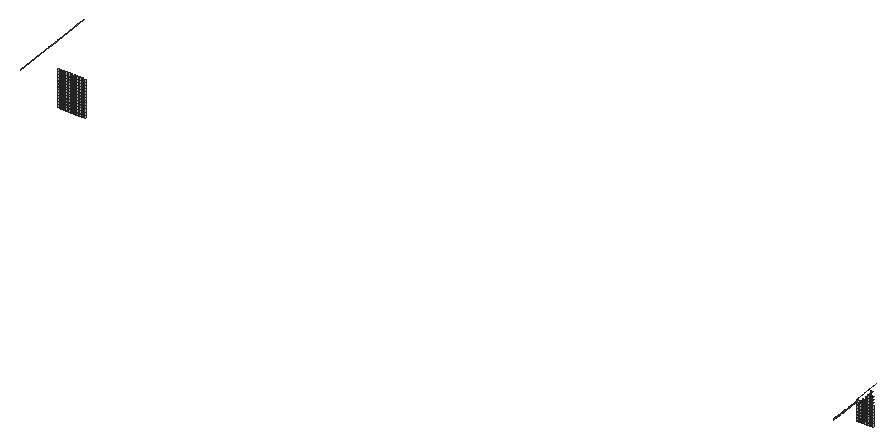
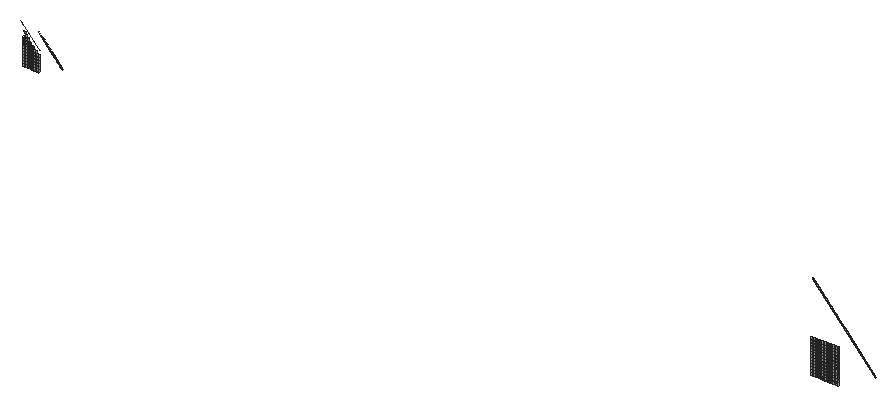
# SketchUp Ruby script. Lengths in inches.
U = 1.inch
M = Sketchup.active_model
def pt(a) = Geom::Point3d.new(a.map { |v| v * U })
def face(e, loops, mat)
  f = e.add_face(loops[0].map { |a| pt(a) })
  loops[1..].each { |l| e.add_face(l.map { |a| pt(a) }).erase! }
  f.material = f.back_material = mat if mat
  f
end
# faces: each face lists its corners as indices into pts; further lists are holes
def faces(e, pts, list, mat = nil) = list.each { |f| face(e, (f[0].is_a?(Array) ? f : [f]).map { |l| l.map { |i| pts[i] } }, mat) }
# xy, xz, yz: faces in a plane at the given z, y or x. An outline is a flat list of corners, or four numbers for a rectangle; further outlines are holes
def ring(l) = l.size == 4 ? [[l[0], l[1]], [l[2], l[1]], [l[2], l[3]], [l[0], l[3]]] : l.each_slice(2).to_a
def flat(e, list, mat, &to3) = list.each { |f| face(e, (f[0].is_a?(Array) ? f : [f]).map { |l| ring(l).map { |u, v| to3.(u, v) } }, mat) }
def xy(e, z, list, mat = nil) = flat(e, list, mat) { |x, y| [x, y, z] }
def xz(e, y, list, mat = nil) = flat(e, list, mat) { |x, z| [x, y, z] }
def yz(e, x, list, mat = nil) = flat(e, list, mat) { |y, z| [x, y, z] }
def lines(e, pts, list) = list.each { |a, b| e.add_line(pt(pts[a]), pt(pts[b])) }
# prism: a flat outline (further loops are holes) pulled along v
def prism(e, loops, v, mat = nil)
  f = face(e, loops, mat); d = Geom::Vector3d.new(v.map { |x| x * U })
  f.pushpull(f.normal.samedirection?(d) ? d.length : -d.length)
end
def box(e, o, s, mat = nil) = prism(e, [[o, [o[0] + s[0], o[1], o[2]], [o[0] + s[0], o[1] + s[1], o[2]], [o[0], o[1] + s[1], o[2]]]], [0, 0, s[2]], mat)
def at(x, y, z, deg = 0) = Geom::Transformation.translation(pt([x, y, z])) * Geom::Transformation.rotation(ORIGIN, Z_AXIS, deg.degrees)
def axes(o, x, y, z) = Geom::Transformation.new([*x, 0, *y, 0, *z, 0, *pt(o).to_a, 1])
def part(name) = M.definitions.add(name)
# library, detail: a bought-in or finely detailed component or shape, given as its bounding box
def library(name, o, s) = part(name).tap { |d| box(d.entities, o, s) }
def detail(e, o, s) = box(e.add_group.entities, o, s)
def put(e, d, t, mat = nil) = e.add_instance(d, t).tap { |i| i.material = mat if mat }
def group(e, t, mat = nil) = e.add_group.tap { |g| g.transformation = t; g.material = mat if mat }.entities
root = M.entities
M.materials.add("[Color M06]").color = [79, 71, 84]
xy(root,305.35,[[1357.49,480.14,1359.8,480.77],[1360.4,480.14,1362.71,480.77],[1363.3125,480.14,1365.625,480.77],[1366.23,480.14,1368.54,480.64],[1369.14,480.14,1371.45,480.64],
  [1372.05,480.14,1374.36,480.64],[1374.96,480.14,1377.27,480.64],[1377.875,480.14,1380.1875,480.77],[1380.79,480.14,1383.1,480.77],[1383.7,480.14,1386.01,480.77],
  [2206.1,480.14,2208.41,480.77],[2209.01,480.14,2211.32,480.77],[2211.92,480.14,2214.23,480.77],[2214.83,480.14,2217.15,480.77],[2217.75,480.14,2220.06,480.77],
  [2220.66,480.14,2222.97,480.77]])
xy(root,307.67,[[1357.49,480.14,1359.8,480.77],[1360.4,480.14,1362.71,480.77],[1363.3125,480.14,1365.625,480.77],[1366.23,480.14,1368.54,480.64],[1369.14,480.14,1371.45,480.64],
  [1372.05,480.14,1374.36,480.64],[1374.96,480.14,1377.27,480.64],[1377.875,480.14,1380.1875,480.77],[1380.79,480.14,1383.1,480.77],[1383.7,480.14,1386.01,480.77],
  [2206.1,480.14,2208.41,480.77],[2209.01,480.14,2211.32,480.77],[2211.92,480.14,2214.23,480.77],[2214.83,480.14,2217.15,480.77],[2217.75,480.14,2220.06,480.77],
  [2220.66,480.14,2222.97,480.77]])
xy(root,308.4,[[1357.52,480.14,1359.83,480.77],[1360.43,480.14,1362.74,480.77],[1363.34,480.14,1365.65,480.77],[1366.25,480.14,1368.57,480.77],[1369.17,480.14,1371.48,480.77],
  [1372.08,480.14,1374.39,480.77],[1374.99,480.14,1377.3,480.77],[1377.9,480.14,1380.22,480.77],[1380.81,480.14,1383.13,480.77],[1383.73,480.14,1386.04,480.77],
  [2206.125,480.14,2208.4375,480.77],[2209.04,480.14,2211.35,480.77],[2211.95,480.14,2214.26,480.77],[2214.86,480.14,2217.17,480.77],[2217.77,480.14,2220.09,480.77],
  [2220.6875,480.14,2223,480.77]])
xy(root,310.71,[[1357.52,480.14,1359.83,480.77],[1360.43,480.14,1362.74,480.77],[1363.34,480.14,1365.65,480.77],[1366.25,480.14,1368.57,480.77],[1369.17,480.14,1371.48,480.77],
  [1372.08,480.14,1374.39,480.77],[1374.99,480.14,1377.3,480.77],[1377.9,480.14,1380.22,480.77],[1380.81,480.14,1383.13,480.77],[1383.73,480.14,1386.04,480.77],
  [2206.125,480.14,2208.4375,480.77],[2209.04,480.14,2211.35,480.77],[2211.95,480.14,2214.26,480.77],[2214.86,480.14,2217.17,480.77],[2217.77,480.14,2220.09,480.77],
  [2220.6875,480.14,2223,480.77]])
xy(root,311.21,[[1357.52,480.14,1359.83,480.77],[1360.43,480.14,1362.74,480.77],[1363.34,480.14,1365.65,480.77],[1366.25,480.14,1368.57,480.77],[1369.17,480.14,1371.48,480.77],
  [1372.08,480.14,1374.39,480.77],[1374.99,480.14,1377.3,480.77],[1377.9,480.14,1380.22,480.77],[1380.81,480.14,1383.13,480.77],[1383.73,480.14,1386.04,480.77],
  [2206.125,480.14,2208.4375,480.77],[2209.04,480.14,2211.35,480.77],[2211.95,480.14,2214.26,480.77],[2214.86,480.14,2217.17,480.77],[2217.77,480.14,2220.09,480.77],
  [2220.6875,480.14,2223,480.77]])
xy(root,313.52,[[1357.52,480.14,1359.83,480.77],[1360.43,480.14,1362.74,480.77],[1363.34,480.14,1365.65,480.77],[1366.25,480.14,1368.57,480.77],[1369.17,480.14,1371.48,480.77],
  [1372.08,480.14,1374.39,480.77],[1374.99,480.14,1377.3,480.77],[1377.9,480.14,1380.22,480.77],[1380.81,480.14,1383.13,480.77],[1383.73,480.14,1386.04,480.77],
  [2206.125,480.14,2208.4375,480.77],[2209.04,480.14,2211.35,480.77],[2211.95,480.14,2214.26,480.77],[2214.86,480.14,2217.17,480.77],[2217.77,480.14,2220.09,480.77],
  [2220.6875,480.14,2223,480.77]])
xy(root,314.02,[[1357.52,480.14,1359.83,480.77],[1360.43,480.14,1362.74,480.77],[1363.34,480.14,1365.65,480.77],[1366.25,480.14,1368.57,480.77],[1369.17,480.14,1371.48,480.77],
  [1372.08,480.14,1374.39,480.77],[1374.99,480.14,1377.3,480.77],[1377.9,480.14,1380.22,480.77],[1380.81,480.14,1383.13,480.77],[1383.73,480.14,1386.04,480.77],
  [2206.125,480.14,2208.4375,480.77],[2209.04,480.14,2211.35,480.77],[2211.95,480.14,2214.26,480.77],[2214.86,480.14,2217.17,480.77],[2217.77,480.14,2220.09,480.77],
  [2220.6875,480.14,2223,480.77]])
xy(root,316.34,[[1357.52,480.14,1359.83,480.77],[1360.43,480.14,1362.74,480.77],[1363.34,480.14,1365.65,480.77],[1366.25,480.14,1368.57,480.77],[1369.17,480.14,1371.48,480.77],
  [1372.08,480.14,1374.39,480.77],[1374.99,480.14,1377.3,480.77],[1377.9,480.14,1380.22,480.77],[1380.81,480.14,1383.13,480.77],[1383.73,480.14,1386.04,480.77],
  [2206.125,480.14,2208.4375,480.77],[2209.04,480.14,2211.35,480.77],[2211.95,480.14,2214.26,480.77],[2214.86,480.14,2217.17,480.77],[2217.77,480.14,2220.09,480.77],
  [2220.6875,480.14,2223,480.77]])
xy(root,316.84,[[1357.52,480.14,1359.83,480.77],[1360.43,480.14,1362.74,480.77],[1363.34,480.14,1365.65,480.77],[1366.25,480.14,1368.57,480.77],[1369.17,480.14,1371.48,480.77],
  [1372.08,480.14,1374.39,480.77],[1374.99,480.14,1377.3,480.77],[1377.9,480.14,1380.22,480.77],[1380.81,480.14,1383.13,480.77],[1383.73,480.14,1386.04,480.77],
  [2206.125,480.14,2208.4375,480.77],[2209.04,480.14,2211.35,480.77],[2211.95,480.14,2214.26,480.77],[2214.86,480.14,2217.17,480.77],[2217.77,480.14,2220.09,480.77],
  [2220.6875,480.14,2223,480.77]])
xy(root,319.15,[[1357.52,480.14,1359.83,480.77],[1360.43,480.14,1362.74,480.77],[1363.34,480.14,1365.65,480.77],[1366.25,480.14,1368.57,480.77],[1369.17,480.14,1371.48,480.77],
  [1372.08,480.14,1374.39,480.77],[1374.99,480.14,1377.3,480.77],[1377.9,480.14,1380.22,480.77],[1380.81,480.14,1383.13,480.77],[1383.73,480.14,1386.04,480.77],
  [2206.125,480.14,2208.4375,480.77],[2209.04,480.14,2211.35,480.77],[2211.95,480.14,2214.26,480.77],[2214.86,480.14,2217.17,480.77],[2217.77,480.14,2220.09,480.77],
  [2220.6875,480.14,2223,480.77]])
xy(root,319.65,[[1357.52,480.14,1359.83,480.77],[1360.43,480.14,1362.74,480.77],[1363.34,480.14,1365.65,480.77],[1366.25,480.14,1368.57,480.77],[1369.17,480.14,1371.48,480.77],
  [1372.08,480.14,1374.39,480.7],[1374.99,480.14,1377.3,480.7],[1377.9,480.14,1380.22,480.7],[1380.81,480.14,1383.13,480.7],[1383.73,480.14,1386.04,480.77],
  [2206.125,480.14,2208.4375,480.77],[2209.04,480.14,2211.35,480.77],[2211.95,480.14,2214.26,480.77],[2214.86,480.14,2217.17,480.77],[2217.77,480.14,2220.09,480.77],
  [2220.6875,480.14,2223,480.77]])
xy(root,321.96,[[1357.52,480.14,1359.83,480.77],[1360.43,480.14,1362.74,480.77],[1363.34,480.14,1365.65,480.77],[1366.25,480.14,1368.57,480.77],[1369.17,480.14,1371.48,480.77],
  [1372.08,480.14,1374.39,480.7],[1374.99,480.14,1377.3,480.7],[1377.9,480.14,1380.22,480.7],[1380.81,480.14,1383.13,480.7],[1383.73,480.14,1386.04,480.77],
  [2206.66,480.14,2208.4375,480.77],[2209.04,480.14,2211.35,480.77],[2211.95,480.14,2214.26,480.77],[2214.86,480.14,2217.17,480.77],[2217.77,480.14,2220.09,480.77],
  [2220.6875,480.14,2223,480.77]])
xy(root,322.46,[[1357.52,480.14,1359.83,480.77],[1360.43,480.14,1362.74,480.77],[1363.34,480.14,1365.65,480.77],[1366.25,480.14,1368.57,480.77],[1369.17,480.14,1371.48,480.77],
  [1372.08,480.14,1374.39,480.77],[1374.99,480.14,1377.3,480.77],[1377.9,480.14,1380.22,480.77],[1380.81,480.14,1383.13,480.77],[1383.73,480.14,1386.04,480.77],
  [2209.04,480.14,2211.35,480.77],[2211.95,480.14,2214.26,480.77],[2214.86,480.14,2217.17,480.77],[2217.77,480.14,2220.09,480.77],[2220.6875,480.14,2223,480.77]])
xy(root,324.77,[[1357.52,480.14,1359.83,480.77],[1360.43,480.14,1362.74,480.77],[1363.34,480.14,1365.65,480.77],[1366.25,480.14,1368.57,480.77],[1369.17,480.14,1371.48,480.77],
  [1372.08,480.14,1374.39,480.77],[1374.99,480.14,1377.3,480.77],[1377.9,480.14,1380.22,480.77],[1380.81,480.14,1383.13,480.77],[1383.73,480.14,1386.04,480.77],
  [2209.29,480.14,2211.35,480.77],[2211.95,480.14,2214.26,480.77],[2214.86,480.14,2217.17,480.77],[2217.77,480.14,2220.09,480.77],[2220.6875,480.14,2223,480.77]])
xy(root,325.27,[[1357.52,480.14,1359.83,480.77],[1360.43,480.14,1362.74,480.77],[1363.34,480.14,1365.65,480.77],[1366.25,480.14,1368.57,480.77],[1369.17,480.14,1371.48,480.77],
  [1372.08,480.14,1374.39,480.77],[1374.99,480.14,1377.3,480.77],[1377.9,480.14,1380.22,480.77],[1380.81,480.14,1383.13,480.77],[1383.73,480.14,1386.04,480.77],
  [2211.95,480.14,2214.26,480.77],[2214.86,480.14,2217.17,480.77],[2217.77,480.14,2220.09,480.77],[2220.6875,480.14,2223,480.77]])
xy(root,327.59,[[1357.52,480.14,1359.83,480.77],[1360.43,480.14,1362.74,480.77],[1363.34,480.14,1365.65,480.77],[1366.25,480.14,1368.57,480.77],[1369.17,480.14,1371.48,480.77],
  [1372.08,480.14,1374.39,480.77],[1374.99,480.14,1377.3,480.77],[1377.9,480.14,1380.22,480.77],[1380.81,480.14,1383.13,480.77],[1383.73,480.14,1386.04,480.77],
  [2211.95,480.14,2214.26,480.77],[2214.86,480.14,2217.17,480.77],[2217.77,480.14,2220.09,480.77],[2220.6875,480.14,2223,480.77]])
xy(root,328.09,[[1357.52,480.14,1359.83,480.77],[1360.43,480.14,1362.74,480.77],[1363.34,480.14,1365.65,480.77],[1366.25,480.14,1368.57,480.77],[1369.17,480.14,1371.48,480.77],
  [1372.08,480.14,1374.39,480.77],[1374.99,480.14,1377.3,480.77],[1377.9,480.14,1380.22,480.77],[1380.81,480.14,1383.13,480.77],[1383.73,480.14,1386.04,480.77],
  [2214.86,480.14,2217.17,480.77],[2217.77,480.14,2220.09,480.77],[2220.6875,480.14,2223,480.77]])
xy(root,330.4,[[1357.52,480.14,1359.83,480.77],[1360.43,480.14,1362.74,480.77],[1363.34,480.14,1365.65,480.77],[1366.25,480.14,1368.57,480.77],[1369.17,480.14,1371.48,480.77],
  [1372.08,480.14,1374.39,480.77],[1374.99,480.14,1377.3,480.77],[1377.9,480.14,1380.22,480.77],[1380.81,480.14,1383.13,480.77],[1383.73,480.14,1386.04,480.77],
  [2214.86,480.14,2217.17,480.77],[2217.77,480.14,2220.09,480.77],[2220.6875,480.14,2223,480.77]])
xy(root,330.9,[[1357.52,480.14,1359.83,480.77],[1360.43,480.14,1362.74,480.77],[1363.34,480.14,1365.65,480.77],[1366.25,480.14,1368.57,480.77],[1369.17,480.14,1371.48,480.77],
  [1372.08,480.14,1374.39,480.77],[1374.99,480.14,1377.3,480.77],[1377.9,480.14,1380.22,480.77],[1380.81,480.14,1383.13,480.77],[1383.73,480.14,1386.04,480.77],
  [2217.77,480.14,2220.09,480.77],[2220.6875,480.14,2223,480.77]])
xy(root,333.21,[[1357.52,480.14,1359.83,480.77],[1360.43,480.14,1362.74,480.77],[1363.34,480.14,1365.65,480.77],[1366.25,480.14,1368.57,480.77],[1369.17,480.14,1371.48,480.77],
  [1372.08,480.14,1374.39,480.77],[1374.99,480.14,1377.3,480.77],[1377.9,480.14,1380.22,480.77],[1380.81,480.14,1383.13,480.77],[1383.73,480.14,1386.04,480.77],
  [2217.77,480.14,2220.09,480.77],[2220.6875,480.14,2223,480.77]])
xy(root,333.71,[[1357.52,480.14,1359.83,480.77],[1360.43,480.14,1362.74,480.77],[1363.34,480.14,1365.65,480.77],[1366.25,480.14,1368.57,480.77],[1369.17,480.14,1371.48,480.77],
  [1372.08,480.14,1374.39,480.77],[1374.99,480.14,1377.3,480.77],[1377.9,480.14,1380.22,480.77],[1380.81,480.14,1383.13,480.77],[1383.73,480.14,1386.04,480.77],
  [2217.77,480.14,2220.09,480.77],[2220.6875,480.14,2223,480.77]])
xy(root,336.02,[[1357.52,480.14,1359.83,480.77],[1360.43,480.14,1362.74,480.77],[1363.34,480.14,1365.65,480.77],[1366.25,480.14,1368.57,480.77],[1369.17,480.14,1371.48,480.77],
  [1372.08,480.14,1374.39,480.77],[1374.99,480.14,1377.3,480.77],[1377.9,480.14,1380.22,480.77],[1380.81,480.14,1383.13,480.77],[1383.73,480.14,1386.04,480.77]])
xy(root,336.52,[[1357.52,480.14,1359.83,480.77],[1360.43,480.14,1362.74,480.77],[1363.34,480.14,1365.65,480.77],[1366.25,480.14,1368.57,480.77],[1369.17,480.14,1371.48,480.77],
  [1372.08,480.14,1374.39,480.77],[1374.99,480.14,1377.3,480.77],[1377.9,480.14,1380.22,480.77],[1380.81,480.14,1383.13,480.77],[1383.73,480.14,1386.04,480.77]])
xy(root,338.84,[[1357.52,480.14,1359.83,480.77],[1360.43,480.14,1362.74,480.77],[1363.34,480.14,1365.65,480.77],[1366.25,480.14,1368.57,480.77],[1369.17,480.14,1371.48,480.77],
  [1372.08,480.14,1374.39,480.77],[1374.99,480.14,1377.3,480.77],[1377.9,480.14,1380.22,480.77],[1380.81,480.14,1383.13,480.77],[1383.73,480.14,1386.04,480.77]])
xy(root,339.34,[[1357.52,480.14,1359.83,480.77],[1360.43,480.14,1362.74,480.77],[1363.34,480.14,1365.65,480.77],[1366.25,480.14,1368.57,480.77],[1369.17,480.14,1371.48,480.77],
  [1372.08,480.14,1374.39,480.77],[1374.99,480.14,1377.3,480.77],[1377.9,480.14,1380.22,480.77],[1380.81,480.14,1383.13,480.77],[1383.73,480.14,1386.04,480.77]])
xz(root,467.1875,[[2192,306.65,2194.42,309.22,2193.96,309.65,2191.54,307.08],[2191.54,307.08,2193.96,309.65,2193.74,309.87,2191.3125,307.29],[2195.3,310.16,2197.72,312.73,2197.26,313.16,2194.84,310.59],[2198.59,313.66,2201.02,316.23,2200.56,316.66,2198.14,314.09],[2201.89,317.17,2204.3125,319.74,2203.86,320.17,2201.4375,317.59],
  [2205.19,320.67,2207.61,323.24,2207.16,323.67,2204.74,321.1],[2208.49,324.17,2210.91,326.75,2210.46,327.17,2208.03,324.6],[2211.79,327.68,2214.21,330.25,2213.75,330.68,2211.33,328.11],[2215.09,331.18,2217.51,333.75,2217.05,334.18,2214.63,331.61]],"[Color M06]")
xz(root,480.14,[[2209.04,324.5,2209.29,324.77,2209.04,324.77],[2220.6875,336.93,2222.47,338.84,2220.6875,338.84]])
yz(root,1356.92,[[480.14,311.21,480.77,313.52],[480.14,314.02,480.77,316.34],[480.14,316.84,480.77,319.15],[480.14,319.65,480.77,321.96],[480.14,322.46,480.77,324.77],
  [480.14,325.27,480.77,327.59],[480.14,328.09,480.77,330.4],[480.14,330.9,480.77,333.21],[480.14,333.71,480.77,336.02],[480.14,336.52,480.77,338.84],
  [480.14,339.34,480.77,341.65]])
yz(root,1357.49,[[480.14,305.35,480.77,307.67]])
yz(root,1357.52,[[480.14,308.4,480.77,310.71],[480.14,311.21,480.77,313.52],[480.14,314.02,480.77,316.34],[480.14,316.84,480.77,319.15],[480.14,319.65,480.77,321.96],
  [480.14,322.46,480.77,324.77],[480.14,325.27,480.77,327.59],[480.14,328.09,480.77,330.4],[480.14,330.9,480.77,333.21],[480.14,333.71,480.77,336.02],
  [480.14,336.52,480.77,338.84],[480.14,339.34,480.77,341.65]])
yz(root,1359.8,[[480.14,305.35,480.77,307.67]])
yz(root,1359.83,[[480.14,308.4,480.77,310.71],[480.14,311.21,480.77,313.52],[480.14,314.02,480.77,316.34],[480.14,316.84,480.77,319.15],[480.14,319.65,480.77,321.96],
  [480.14,322.46,480.77,324.77],[480.14,325.27,480.77,327.59],[480.14,328.09,480.77,330.4],[480.14,330.9,480.77,333.21],[480.14,333.71,480.77,336.02],
  [480.14,336.52,480.77,338.84],[480.14,339.34,480.77,341.65]])
yz(root,1360.4,[[480.14,305.35,480.77,307.67]])
yz(root,1360.43,[[480.14,308.4,480.77,310.71],[480.14,311.21,480.77,313.52],[480.14,314.02,480.77,316.34],[480.14,316.84,480.77,319.15],[480.14,319.65,480.77,321.96],
  [480.14,322.46,480.77,324.77],[480.14,325.27,480.77,327.59],[480.14,328.09,480.77,330.4],[480.14,330.9,480.77,333.21],[480.14,333.71,480.77,336.02],
  [480.14,336.52,480.77,338.84],[480.14,339.34,480.77,341.65]])
yz(root,1362.71,[[480.14,305.35,480.77,307.67]])
yz(root,1362.74,[[480.14,308.4,480.77,310.71],[480.14,311.21,480.77,313.52],[480.14,314.02,480.77,316.34],[480.14,316.84,480.77,319.15],[480.14,319.65,480.77,321.96],
  [480.14,322.46,480.77,324.77],[480.14,325.27,480.77,327.59],[480.14,328.09,480.77,330.4],[480.14,330.9,480.77,333.21],[480.14,333.71,480.77,336.02],
  [480.14,336.52,480.77,338.84],[480.14,339.34,480.77,341.65]])
yz(root,1363.3125,[[480.14,305.35,480.77,307.67]])
yz(root,1363.34,[[480.14,308.4,480.77,310.71],[480.14,311.21,480.77,313.52],[480.14,314.02,480.77,316.34],[480.14,316.84,480.77,319.15],[480.14,319.65,480.77,321.96],
  [480.14,322.46,480.77,324.77],[480.14,325.27,480.77,327.59],[480.14,328.09,480.77,330.4],[480.14,330.9,480.77,333.21],[480.14,333.71,480.77,336.02],
  [480.14,336.52,480.77,338.84],[480.14,339.34,480.77,341.65]])
yz(root,1365.625,[[480.14,305.35,480.77,307.67]])
yz(root,1365.65,[[480.14,308.4,480.77,310.71],[480.14,311.21,480.77,313.52],[480.14,314.02,480.77,316.34],[480.14,316.84,480.77,319.15],[480.14,319.65,480.77,321.96],
  [480.14,322.46,480.77,324.77],[480.14,325.27,480.77,327.59],[480.14,328.09,480.77,330.4],[480.14,330.9,480.77,333.21],[480.14,333.71,480.77,336.02],
  [480.14,336.52,480.77,338.84],[480.14,339.34,480.77,341.65]])
yz(root,1366.23,[[480.14,305.35,480.64,307.67]])
yz(root,1366.25,[[480.14,308.4,480.77,310.71],[480.14,311.21,480.77,313.52],[480.14,314.02,480.77,316.34],[480.14,316.84,480.77,319.15],[480.14,319.65,480.77,321.96],
  [480.14,322.46,480.77,324.77],[480.14,325.27,480.77,327.59],[480.14,328.09,480.77,330.4],[480.14,330.9,480.77,333.21],[480.14,333.71,480.77,336.02],
  [480.14,336.52,480.77,338.84],[480.14,339.34,480.77,341.65]])
yz(root,1368.54,[[480.14,305.35,480.64,307.67]])
yz(root,1368.57,[[480.14,308.4,480.77,310.71],[480.14,311.21,480.77,313.52],[480.14,314.02,480.77,316.34],[480.14,316.84,480.77,319.15],[480.14,319.65,480.77,321.96],
  [480.14,322.46,480.77,324.77],[480.14,325.27,480.77,327.59],[480.14,328.09,480.77,330.4],[480.14,330.9,480.77,333.21],[480.14,333.71,480.77,336.02],
  [480.14,336.52,480.77,338.84],[480.14,339.34,480.77,341.65]])
yz(root,1369.14,[[480.14,305.35,480.64,307.67]])
yz(root,1369.17,[[480.14,308.4,480.77,310.71],[480.14,311.21,480.77,313.52],[480.14,314.02,480.77,316.34],[480.14,316.84,480.77,319.15],[480.14,319.65,480.77,321.96],
  [480.14,322.46,480.77,324.77],[480.14,325.27,480.77,327.59],[480.14,328.09,480.77,330.4],[480.14,330.9,480.77,333.21],[480.14,333.71,480.77,336.02],
  [480.14,336.52,480.77,338.84],[480.14,339.34,480.77,341.65]])
yz(root,1371.45,[[480.14,305.35,480.64,307.67]])
yz(root,1371.48,[[480.14,308.4,480.77,310.71],[480.14,311.21,480.77,313.52],[480.14,314.02,480.77,316.34],[480.14,316.84,480.77,319.15],[480.14,319.65,480.77,321.96],
  [480.14,322.46,480.77,324.77],[480.14,325.27,480.77,327.59],[480.14,328.09,480.77,330.4],[480.14,330.9,480.77,333.21],[480.14,333.71,480.77,336.02],
  [480.14,336.52,480.77,338.84],[480.14,339.34,480.77,341.65]])
yz(root,1372.05,[[480.14,305.35,480.64,307.67]])
yz(root,1372.08,[[480.14,308.4,480.77,310.71],[480.14,311.21,480.77,313.52],[480.14,314.02,480.77,316.34],[480.14,316.84,480.77,319.15],[480.14,319.65,480.7,321.96],
  [480.14,322.46,480.77,324.77],[480.14,325.27,480.77,327.59],[480.14,328.09,480.77,330.4],[480.14,330.9,480.77,333.21],[480.14,333.71,480.77,336.02],
  [480.14,336.52,480.77,338.84],[480.14,339.34,480.77,341.65]])
yz(root,1374.36,[[480.14,305.35,480.64,307.67]])
yz(root,1374.39,[[480.14,308.4,480.77,310.71],[480.14,311.21,480.77,313.52],[480.14,314.02,480.77,316.34],[480.14,316.84,480.77,319.15],[480.14,319.65,480.7,321.96],
  [480.14,322.46,480.77,324.77],[480.14,325.27,480.77,327.59],[480.14,328.09,480.77,330.4],[480.14,330.9,480.77,333.21],[480.14,333.71,480.77,336.02],
  [480.14,336.52,480.77,338.84],[480.14,339.34,480.77,341.65]])
yz(root,1374.96,[[480.14,305.35,480.64,307.67]])
yz(root,1374.99,[[480.14,308.4,480.77,310.71],[480.14,311.21,480.77,313.52],[480.14,314.02,480.77,316.34],[480.14,316.84,480.77,319.15],[480.14,319.65,480.7,321.96],
  [480.14,322.46,480.77,324.77],[480.14,325.27,480.77,327.59],[480.14,328.09,480.77,330.4],[480.14,330.9,480.77,333.21],[480.14,333.71,480.77,336.02],
  [480.14,336.52,480.77,338.84],[480.14,339.34,480.77,341.65]])
yz(root,1377.27,[[480.14,305.35,480.64,307.67]])
yz(root,1377.3,[[480.14,308.4,480.77,310.71],[480.14,311.21,480.77,313.52],[480.14,314.02,480.77,316.34],[480.14,316.84,480.77,319.15],[480.14,319.65,480.7,321.96],
  [480.14,322.46,480.77,324.77],[480.14,325.27,480.77,327.59],[480.14,328.09,480.77,330.4],[480.14,330.9,480.77,333.21],[480.14,333.71,480.77,336.02],
  [480.14,336.52,480.77,338.84],[480.14,339.34,480.77,341.65]])
yz(root,1377.875,[[480.14,305.35,480.77,307.67]])
yz(root,1377.9,[[480.14,308.4,480.77,310.71],[480.14,311.21,480.77,313.52],[480.14,314.02,480.77,316.34],[480.14,316.84,480.77,319.15],[480.14,319.65,480.7,321.96],
  [480.14,322.46,480.77,324.77],[480.14,325.27,480.77,327.59],[480.14,328.09,480.77,330.4],[480.14,330.9,480.77,333.21],[480.14,333.71,480.77,336.02],
  [480.14,336.52,480.77,338.84],[480.14,339.34,480.77,341.65]])
yz(root,1380.1875,[[480.14,305.35,480.77,307.67]])
yz(root,1380.22,[[480.14,308.4,480.77,310.71],[480.14,311.21,480.77,313.52],[480.14,314.02,480.77,316.34],[480.14,316.84,480.77,319.15],[480.14,319.65,480.7,321.96],
  [480.14,322.46,480.77,324.77],[480.14,325.27,480.77,327.59],[480.14,328.09,480.77,330.4],[480.14,330.9,480.77,333.21],[480.14,333.71,480.77,336.02],
  [480.14,336.52,480.77,338.84],[480.14,339.34,480.77,341.65]])
yz(root,1380.79,[[480.14,305.35,480.77,307.67]])
yz(root,1380.81,[[480.14,308.4,480.77,310.71],[480.14,311.21,480.77,313.52],[480.14,314.02,480.77,316.34],[480.14,316.84,480.77,319.15],[480.14,319.65,480.7,321.96],
  [480.14,322.46,480.77,324.77],[480.14,325.27,480.77,327.59],[480.14,328.09,480.77,330.4],[480.14,330.9,480.77,333.21],[480.14,333.71,480.77,336.02],
  [480.14,336.52,480.77,338.84],[480.14,339.34,480.77,341.65]])
yz(root,1383.1,[[480.14,305.35,480.77,307.67]])
yz(root,1383.13,[[480.14,308.4,480.77,310.71],[480.14,311.21,480.77,313.52],[480.14,314.02,480.77,316.34],[480.14,316.84,480.77,319.15],[480.14,319.65,480.7,321.96],
  [480.14,322.46,480.77,324.77],[480.14,325.27,480.77,327.59],[480.14,328.09,480.77,330.4],[480.14,330.9,480.77,333.21],[480.14,333.71,480.77,336.02],
  [480.14,336.52,480.77,338.84],[480.14,339.34,480.77,341.65]])
yz(root,1383.7,[[480.14,305.35,480.77,307.67]])
yz(root,1383.73,[[480.14,308.4,480.77,310.71],[480.14,311.21,480.77,313.52],[480.14,314.02,480.77,316.34],[480.14,316.84,480.77,319.15],[480.14,319.65,480.77,321.96],
  [480.14,322.46,480.77,324.77],[480.14,325.27,480.77,327.59],[480.14,328.09,480.77,330.4],[480.14,330.9,480.77,333.21],[480.14,333.71,480.77,336.02],
  [480.14,336.52,480.77,338.84],[480.14,339.34,480.77,341.65]])
yz(root,1386.01,[[480.14,305.35,480.77,307.67]])
yz(root,1386.04,[[480.14,308.4,480.77,310.71],[480.14,311.21,480.77,313.52],[480.14,314.02,480.77,316.34],[480.14,316.84,480.77,319.15],[480.14,319.65,480.77,321.96],
  [480.14,322.46,480.77,324.77],[480.14,325.27,480.77,327.59],[480.14,328.09,480.77,330.4],[480.14,330.9,480.77,333.21],[480.14,333.71,480.77,336.02],
  [480.14,336.52,480.77,338.84],[480.14,339.34,480.77,341.65]])
yz(root,2206.1,[[480.14,305.35,480.77,307.67]])
yz(root,2206.125,[[480.14,308.4,480.77,310.71],[480.14,311.21,480.77,313.52],[480.14,314.02,480.77,316.34],[480.14,316.84,480.77,319.15],[480.14,319.65,480.77,321.39]])
yz(root,2208.41,[[480.14,305.35,480.77,307.67]])
yz(root,2208.4375,[[480.14,308.4,480.77,310.71],[480.14,311.21,480.77,313.52],[480.14,314.02,480.77,316.34],[480.14,316.84,480.77,319.15],[480.14,319.65,480.77,321.96]])
yz(root,2209.01,[[480.14,305.35,480.77,307.67]])
yz(root,2209.04,[[480.14,308.4,480.77,310.71],[480.14,311.21,480.77,313.52],[480.14,314.02,480.77,316.34],[480.14,316.84,480.77,319.15],[480.14,319.65,480.77,321.96],
  [480.14,322.46,480.77,324.5]])
yz(root,2211.32,[[480.14,305.35,480.77,307.67]])
yz(root,2211.35,[[480.14,308.4,480.77,310.71],[480.14,311.21,480.77,313.52],[480.14,314.02,480.77,316.34],[480.14,316.84,480.77,319.15],[480.14,319.65,480.77,321.96],
  [480.14,322.46,480.77,324.77]])
yz(root,2211.92,[[480.14,305.35,480.77,307.67]])
yz(root,2211.95,[[480.14,308.4,480.77,310.71],[480.14,311.21,480.77,313.52],[480.14,314.02,480.77,316.34],[480.14,316.84,480.77,319.15],[480.14,319.65,480.77,321.96],
  [480.14,322.46,480.77,324.77],[480.14,325.27,480.77,327.59]])
yz(root,2214.23,[[480.14,305.35,480.77,307.67]])
yz(root,2214.26,[[480.14,308.4,480.77,310.71],[480.14,311.21,480.77,313.52],[480.14,314.02,480.77,316.34],[480.14,316.84,480.77,319.15],[480.14,319.65,480.77,321.96],
  [480.14,322.46,480.77,324.77],[480.14,325.27,480.77,327.59]])
yz(root,2214.83,[[480.14,305.35,480.77,307.67]])
yz(root,2214.86,[[480.14,308.4,480.77,310.71],[480.14,311.21,480.77,313.52],[480.14,314.02,480.77,316.34],[480.14,316.84,480.77,319.15],[480.14,319.65,480.77,321.96],
  [480.14,322.46,480.77,324.77],[480.14,325.27,480.77,327.59],[480.14,328.09,480.77,330.4]])
yz(root,2217.15,[[480.14,305.35,480.77,307.67]])
yz(root,2217.17,[[480.14,308.4,480.77,310.71],[480.14,311.21,480.77,313.52],[480.14,314.02,480.77,316.34],[480.14,316.84,480.77,319.15],[480.14,319.65,480.77,321.96],
  [480.14,322.46,480.77,324.77],[480.14,325.27,480.77,327.59],[480.14,328.09,480.77,330.4]])
yz(root,2217.75,[[480.14,305.35,480.77,307.67]])
yz(root,2217.77,[[480.14,308.4,480.77,310.71],[480.14,311.21,480.77,313.52],[480.14,314.02,480.77,316.34],[480.14,316.84,480.77,319.15],[480.14,319.65,480.77,321.96],
  [480.14,322.46,480.77,324.77],[480.14,325.27,480.77,327.59],[480.14,328.09,480.77,330.4],[480.14,330.9,480.77,333.21],[480.14,333.71,480.77,333.82]])
yz(root,2220.06,[[480.14,305.35,480.77,307.67]])
yz(root,2220.09,[[480.14,308.4,480.77,310.71],[480.14,311.21,480.77,313.52],[480.14,314.02,480.77,316.34],[480.14,316.84,480.77,319.15],[480.14,319.65,480.77,321.96],
  [480.14,322.46,480.77,324.77],[480.14,325.27,480.77,327.59],[480.14,328.09,480.77,330.4],[480.14,330.9,480.77,333.21],[480.14,333.71,480.77,336.02]])
yz(root,2220.66,[[480.14,305.35,480.77,307.67]])
yz(root,2220.6875,[[480.14,308.4,480.77,310.71],[480.14,311.21,480.77,313.52],[480.14,314.02,480.77,316.34],[480.14,316.84,480.77,319.15],[480.14,319.65,480.77,321.96],
  [480.14,322.46,480.77,324.77],[480.14,325.27,480.77,327.59],[480.14,328.09,480.77,330.4],[480.14,330.9,480.77,333.21],[480.14,333.71,480.77,336.02]])
yz(root,2222.97,[[480.14,305.35,480.77,307.67]])
yz(root,2223,[[480.14,308.4,480.77,310.71],[480.14,311.21,480.77,313.52],[480.14,314.02,480.77,316.34],[480.14,316.84,480.77,319.15],[480.14,319.65,480.77,321.96],
  [480.14,322.46,480.77,324.77]])
p = [[2206.66,480.14,321.96],[2206.125,480.14,321.39],[2206.125,480.77,321.39],[2206.66,480.77,321.96],[2209.29,480.14,324.77],[2209.04,480.14,324.5],
  [2209.04,480.77,324.5],[2209.29,480.77,324.77],[1378.99,480.14,391.9],[1384.5,480.14,397.75],[1384.5,480.77,397.75],[1317.4375,480.77,326.5],
  [1317.4375,480.14,326.5],[1340.11,480.14,350.59],[1342.28,480.14,352.9],[1342.96,480.14,353.62],[1344.93,480.14,355.71],[1345.87,480.14,356.71],
  [1347.58,480.14,358.52],[1348.05,480.14,359.02],[1348.18,480.14,359.17],[1348.78,480.14,359.8],[1350.23,480.14,361.34],[1350.7,480.14,361.84],
  [1351.09,480.14,362.26],[1351.69,480.14,362.9],[1352.875,480.14,364.15],[1353.34,480.14,364.65],[1354.01,480.14,365.35],[1354.61,480.14,365.99],
  [1355.52,480.14,366.96],[1355.99,480.14,367.46],[1356.92,480.14,368.45],[1357.52,480.14,369.08],[1358.17,480.14,369.77],[1358.64,480.14,370.27],
  [1359.83,480.14,371.54],[1360.43,480.14,372.18],[1360.82,480.14,372.59],[1361.29,480.14,373.09],[1362.74,480.14,374.63],[1363.34,480.14,375.27],
  [1363.46,480.14,375.4],[1363.875,480.14,375.84],[1365.65,480.14,377.73],[1366.46,480.14,378.59],[1368.57,480.14,380.82],[1369.17,480.14,381.46],
  [1371.23,480.14,383.65],[1372.08,480.14,384.55],[1373.82,480.14,386.4],[1374.23,480.14,386.84],[1374.39,480.14,387.01],[1374.99,480.14,387.65],
  [1376.41,480.14,389.15],[1376.82,480.14,389.59],[1377.3,480.14,390.1],[1377.9,480.14,390.74],[2226.52,480.14,347.77],[2205.79,480.14,325.75]]
faces(root,p,[[0,1,2,3],[4,5,6,7],[8,9,10,11,12,13,14,15,16,17,18,19,20,21,22,23,24,25,26,27,28,29,30,31,32,33,34,35,36,37,38,39,40,41,42,43,44,45,46,47,48,49,50,51,52,53,54,55,56,57]])
lines(root,p,[[58,59]])
